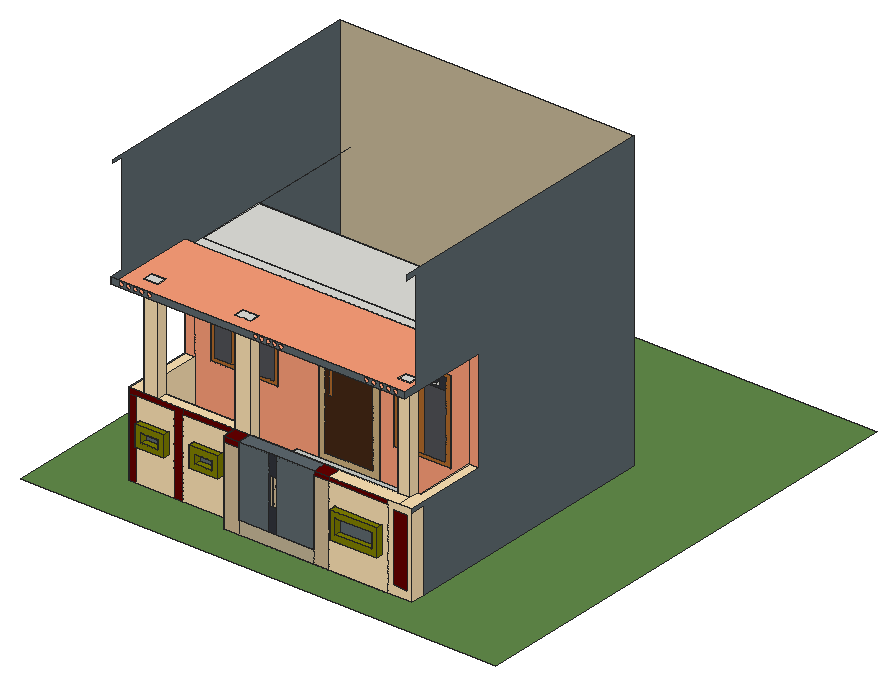
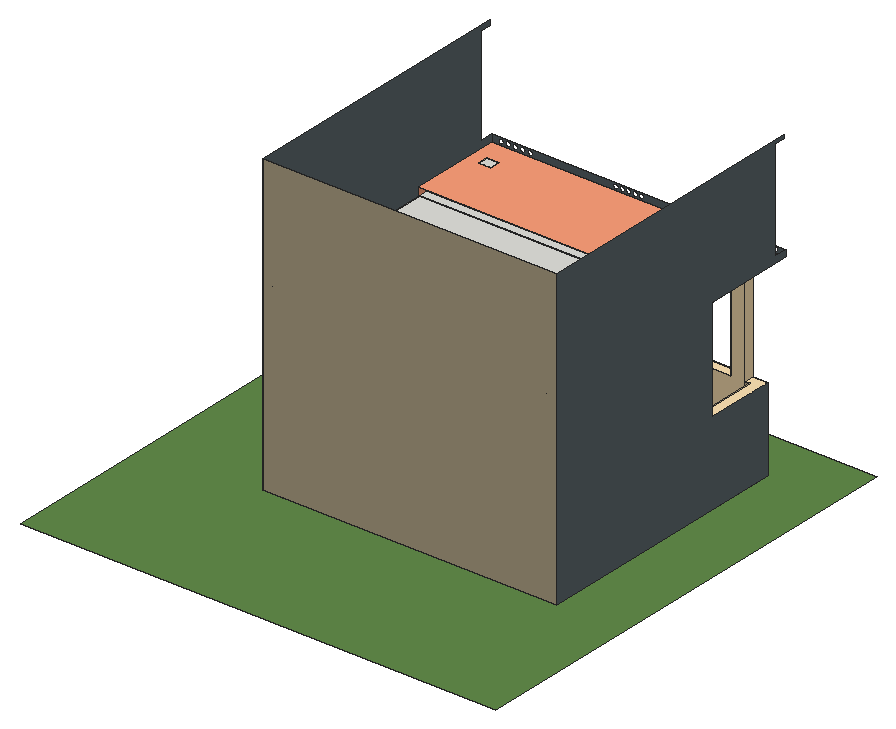
# SketchUp Ruby script. Lengths in inches.
U = 1.inch
M = Sketchup.active_model
def pt(a) = Geom::Point3d.new(a.map { |v| v * U })
def face(e, loops, mat)
  f = e.add_face(loops[0].map { |a| pt(a) })
  loops[1..].each { |l| e.add_face(l.map { |a| pt(a) }).erase! }
  f.material = f.back_material = mat if mat
  f
end
# faces: each face lists its corners as indices into pts; further lists are holes
def faces(e, pts, list, mat = nil) = list.each { |f| face(e, (f[0].is_a?(Array) ? f : [f]).map { |l| l.map { |i| pts[i] } }, mat) }
# xy, xz, yz: faces in a plane at the given z, y or x. An outline is a flat list of corners, or four numbers for a rectangle; further outlines are holes
def ring(l) = l.size == 4 ? [[l[0], l[1]], [l[2], l[1]], [l[2], l[3]], [l[0], l[3]]] : l.each_slice(2).to_a
def flat(e, list, mat, &to3) = list.each { |f| face(e, (f[0].is_a?(Array) ? f : [f]).map { |l| ring(l).map { |u, v| to3.(u, v) } }, mat) }
def xy(e, z, list, mat = nil) = flat(e, list, mat) { |x, y| [x, y, z] }
def xz(e, y, list, mat = nil) = flat(e, list, mat) { |x, z| [x, y, z] }
def yz(e, x, list, mat = nil) = flat(e, list, mat) { |y, z| [x, y, z] }
def lines(e, pts, list) = list.each { |a, b| e.add_line(pt(pts[a]), pt(pts[b])) }
# prism: a flat outline (further loops are holes) pulled along v
def prism(e, loops, v, mat = nil)
  f = face(e, loops, mat); d = Geom::Vector3d.new(v.map { |x| x * U })
  f.pushpull(f.normal.samedirection?(d) ? d.length : -d.length)
end
def box(e, o, s, mat = nil) = prism(e, [[o, [o[0] + s[0], o[1], o[2]], [o[0] + s[0], o[1] + s[1], o[2]], [o[0], o[1] + s[1], o[2]]]], [0, 0, s[2]], mat)
def at(x, y, z, deg = 0) = Geom::Transformation.translation(pt([x, y, z])) * Geom::Transformation.rotation(ORIGIN, Z_AXIS, deg.degrees)
def axes(o, x, y, z) = Geom::Transformation.new([*x, 0, *y, 0, *z, 0, *pt(o).to_a, 1])
def part(name) = M.definitions.add(name)
# library, detail: a bought-in or finely detailed component or shape, given as its bounding box
def library(name, o, s) = part(name).tap { |d| box(d.entities, o, s) }
def detail(e, o, s) = box(e.add_group.entities, o, s)
def put(e, d, t, mat = nil) = e.add_instance(d, t).tap { |i| i.material = mat if mat }
def group(e, t, mat = nil) = e.add_group.tap { |g| g.transformation = t; g.material = mat if mat }.entities
root = M.entities
M.materials.add("[0022_Maroon]").color = [128, 0, 0]
M.materials.add("[0026_LightSalmon]").color = [255, 160, 122]
M.materials.add("[0032_Moccasin]").color = [255, 228, 181]
M.materials.add("[0058_Olive]").color = [128, 128, 0]
M.materials.add("[Basic Tile]").color = [203, 206, 202]
M.materials.add("[Blinds Roman Hobbled Blue]").color = [81, 82, 87]
M.materials.add("[Carpet Berber Pattern Gray]").color = [165, 165, 165]
M.materials.add("[Color A08]").color = [102, 0, 0]
M.materials.add("[Color E08]").color = [102, 102, 0]
M.materials.add("[Formica Beige]").color = [211, 187, 149]
M.materials.add("[Formica Graystone]").color = [149, 146, 135]
M.materials.add("[Formica Laminate Dark]").color = [50, 53, 60]
M.materials.add("[Formica Speckled Grey]").color = [94, 105, 111]
M.materials.add("[Leather Blue]").color = [45, 57, 74]
M.materials.add("[Quartz Light Brown]").color = [199, 184, 152]
M.materials.add("[Terrazzo Light Blue]").color = [196, 214, 227]
M.materials.add("[Vegetation Grass Artificial]").color = [98, 140, 74]
M.materials.add("[Wood Bamboo]").color = [177, 105, 43]
M.materials.add("[Wood Floor Light]").color = [204, 176, 127]
M.materials.add("[Wood Veneer 01]").color = [68, 40, 21]
xy(root,0,[[120.55,26.1,120.55,35.67,47,35.67,47,218.93,251.02,218.93,251.02,35.67,233.76,35.67,233.76,26.1],[233.76,26.1,251.02,35.67]])
xy(root,0,[[0,0,330.1875,330.1875]],"[Vegetation Grass Artificial]")
xy(root,9,[[130.89,26.1,183.14,35.67],[53.84,91.2,244.18,139.9]])
xy(root,9,[[131.52,35.67,233.76,42.51]],"[Carpet Berber Pattern Gray]")
xy(root,9,[[53.84,42.51,244.18,42.51,244.18,84.33,199.57,84.33,199.57,53.64,124.76,53.64,124.76,84.33,53.84,84.33]],"[Leather Blue]")
xy(root,16.4375,[[124.76,53.64,199.57,63.72]],"[Basic Tile]")
xy(root,20.375,[[124.76,63.72,199.57,73.8]],"[Basic Tile]")
xy(root,22.07,[[197.18,21.79,230.37,26.1]],"[0058_Olive]")
xy(root,25.48,[[54.61,31.1,74.79,35.67],[91.98,31.1,112.17,35.67]],"[0058_Olive]")
xy(root,25.78,[[139.85,84.33,181.85,91.2]])
xy(root,25.78,[[124.76,73.8,199.57,84.33]],"[Basic Tile]")
xy(root,26.13,[[201.24,21.79,226.3,26.1]],"[0058_Olive]")
xy(root,29.55,[[58.67,31.1,70.73,35.67],[96.05,31.1,108.1,35.67]],"[0058_Olive]")
xy(root,35.79,[[58.67,31.1,70.73,35.67],[96.05,31.1,108.1,35.67]],"[0058_Olive]")
xy(root,36.69,[[201.24,21.79,226.3,26.1]],"[0058_Olive]")
xy(root,39.86,[[54.61,31.1,74.79,35.67],[91.98,31.1,112.17,35.67]],"[0058_Olive]")
xy(root,40.75,[[197.18,21.79,230.37,26.1]],"[0058_Olive]")
xy(root,50.11,[[192.03,84.33,231.1,91.2]])
xy(root,57.875,[[193.46,26.1,241.9375,35.67],[241.9375,26.1,251.02,26.1,251.02,84.33,244.18,84.33,244.18,42.51,241.9375,42.51],[47,35.67,56.97,35.67,56.97,42.51,53.84,42.51,53.84,84.33,47,84.33],[66.79,35.67,120.55,42.51]],"[0032_Moccasin]")
xy(root,57.875,[[120.55,26.1,130.89,35.67],[183.14,26.1,193.46,35.67]],"[Color A08]")
xy(root,57.875,[[130.89,26.1,183.14,35.67]],"[Formica Speckled Grey]")
xy(root,59.35,[[64.57,84.33,111.51,91.2]])
xy(root,109.17,[[192.03,84.33,231.1,91.2]])
xy(root,113.17,[[64.57,84.33,111.51,91.2]])
xy(root,119.59,[[139.85,84.33,181.85,91.2]])
xy(root,129,[[56.97,35.67,66.79,42.51],[120.55,35.67,131.52,42.51],[233.76,35.67,241.9375,42.51],[53.84,84.33,244.18,91.2],[53.84,91.2,244.18,139.9]])
xy(root,129,[[[47,20.01,251.02,84.33],[120.55,35.67,131.52,42.51],[56.97,35.67,66.79,42.51],[233.76,35.67,241.9375,42.51]]],"[0026_LightSalmon]")
xz(root,20.01,[[[47,129,251.02,133.625],[244.56,129.67,244.09,129.73,243.65,129.91,243.28,130.2,242.99,130.57,242.81,131.01,242.75,131.48,242.81,131.95,242.99,132.38,243.28,132.76,243.65,133.05,244.09,133.23,244.56,133.29,245.03,133.23,245.47,133.05,245.84,132.76,246.13,132.38,246.3125,131.95,246.37,131.48,246.3125,131.01,246.13,130.57,245.84,130.2,245.47,129.91,245.03,129.73],[239.62,129.67,239.15,129.73,238.72,129.91,238.34,130.2,238.05,130.57,237.87,131.01,237.81,131.48,237.87,131.95,238.05,132.38,238.34,132.76,238.72,133.05,239.15,133.23,239.62,133.29,240.09,133.23,240.53,133.05,240.9,132.76,241.19,132.38,241.375,131.95,241.44,131.48,241.375,131.01,241.19,130.57,240.9,130.2,240.53,129.91,240.09,129.73],[234.56,129.67,234.09,129.73,233.65,129.91,233.28,130.2,232.99,130.57,232.81,131.01,232.75,131.48,232.81,131.95,232.99,132.38,233.28,132.76,233.65,133.05,234.09,133.23,234.56,133.29,235.03,133.23,235.47,133.05,235.84,132.76,236.13,132.38,236.3125,131.95,236.37,131.48,236.3125,131.01,236.13,130.57,235.84,130.2,235.47,129.91,235.03,129.73],[229.44,129.67,228.97,129.73,228.53,129.91,228.15,130.2,227.87,130.57,227.68,131.01,227.62,131.48,227.68,131.95,227.87,132.38,228.15,132.76,228.53,133.05,228.97,133.23,229.44,133.29,229.9,133.23,230.34,133.05,230.72,132.76,231,132.38,231.1875,131.95,231.25,131.48,231.1875,131.01,231,130.57,230.72,130.2,230.34,129.91,229.9,129.73],[224.19,129.67,223.72,129.73,223.28,129.91,222.9,130.2,222.62,130.57,222.43,131.01,222.37,131.48,222.43,131.95,222.62,132.38,222.9,132.76,223.28,133.05,223.72,133.23,224.19,133.29,224.65,133.23,225.09,133.05,225.47,132.76,225.75,132.38,225.9375,131.95,226,131.48,225.9375,131.01,225.75,130.57,225.47,130.2,225.09,129.91,224.65,129.73],[58.94,129.67,58.47,129.73,58.03,129.91,57.65,130.2,57.37,130.57,57.18,131.01,57.12,131.48,57.18,131.95,57.37,132.38,57.65,132.76,58.03,133.05,58.47,133.23,58.94,133.29,59.4,133.23,59.84,133.05,60.22,132.76,60.5,132.38,60.6875,131.95,60.75,131.48,60.6875,131.01,60.5,130.57,60.22,130.2,59.84,129.91,59.4,129.73],[63.56,129.67,63.09,129.73,62.65,129.91,62.28,130.2,61.99,130.57,61.81,131.01,61.75,131.48,61.81,131.95,61.99,132.38,62.28,132.76,62.65,133.05,63.09,133.23,63.56,133.29,64.03,133.23,64.47,133.05,64.84,132.76,65.13,132.38,65.3125,131.95,65.37,131.48,65.3125,131.01,65.13,130.57,64.84,130.2,64.47,129.91,64.03,129.73],[68.31,129.67,67.84,129.73,67.4,129.91,67.03,130.2,66.74,130.57,66.56,131.01,66.5,131.48,66.56,131.95,66.74,132.38,67.03,132.76,67.4,133.05,67.84,133.23,68.31,133.29,68.78,133.23,69.22,133.05,69.59,132.76,69.88,132.38,70.0625,131.95,70.12,131.48,70.0625,131.01,69.88,130.57,69.59,130.2,69.22,129.91,68.78,129.73],[73.62,129.67,73.15,129.73,72.72,129.91,72.34,130.2,72.05,130.57,71.87,131.01,71.81,131.48,71.87,131.95,72.05,132.38,72.34,132.76,72.72,133.05,73.15,133.23,73.62,133.29,74.09,133.23,74.53,133.05,74.9,132.76,75.19,132.38,75.375,131.95,75.44,131.48,75.375,131.01,75.19,130.57,74.9,130.2,74.53,129.91,74.09,129.73],[147.06,129.67,146.59,129.73,146.15,129.91,145.78,130.2,145.49,130.57,145.31,131.01,145.25,131.48,145.31,131.95,145.49,132.38,145.78,132.76,146.15,133.05,146.59,133.23,147.06,133.29,147.53,133.23,147.97,133.05,148.34,132.76,148.63,132.38,148.8125,131.95,148.87,131.48,148.8125,131.01,148.63,130.57,148.34,130.2,147.97,129.91,147.53,129.73],[151.44,129.67,150.97,129.73,150.53,129.91,150.15,130.2,149.87,130.57,149.68,131.01,149.62,131.48,149.68,131.95,149.87,132.38,150.15,132.76,150.53,133.05,150.97,133.23,151.44,133.29,151.9,133.23,152.34,133.05,152.72,132.76,153,132.38,153.1875,131.95,153.25,131.48,153.1875,131.01,153,130.57,152.72,130.2,152.34,129.91,151.9,129.73],[156,129.67,155.53,129.73,155.09,129.91,154.72,130.2,154.43,130.57,154.25,131.01,154.19,131.48,154.25,131.95,154.43,132.38,154.72,132.76,155.09,133.05,155.53,133.23,156,133.29,156.47,133.23,156.9,133.05,157.28,132.76,157.57,132.38,157.75,131.95,157.81,131.48,157.75,131.01,157.57,130.57,157.28,130.2,156.9,129.91,156.47,129.73],[160.31,129.67,159.84,129.73,159.4,129.91,159.03,130.2,158.74,130.57,158.56,131.01,158.5,131.48,158.56,131.95,158.74,132.38,159.03,132.76,159.4,133.05,159.84,133.23,160.31,133.29,160.78,133.23,161.22,133.05,161.59,132.76,161.88,132.38,162.0625,131.95,162.12,131.48,162.0625,131.01,161.88,130.57,161.59,130.2,161.22,129.91,160.78,129.73],[164.87,129.67,164.4,129.73,163.97,129.91,163.59,130.2,163.3,130.57,163.12,131.01,163.06,131.48,163.12,131.95,163.3,132.38,163.59,132.76,163.97,133.05,164.4,133.23,164.87,133.29,165.34,133.23,165.78,133.05,166.15,132.76,166.44,132.38,166.625,131.95,166.69,131.48,166.625,131.01,166.44,130.57,166.15,130.2,165.78,129.91,165.34,129.73],[54,129.67,53.53,129.73,53.09,129.91,52.72,130.2,52.43,130.57,52.25,131.01,52.19,131.48,52.25,131.95,52.43,132.38,52.72,132.76,53.09,133.05,53.53,133.23,54,133.29,54.47,133.23,54.9,133.05,55.28,132.76,55.57,132.38,55.75,131.95,55.81,131.48,55.75,131.01,55.57,130.57,55.28,130.2,54.9,129.91,54.47,129.73]]],"[Formica Speckled Grey]")
xz(root,21.79,[[[197.18,22.07,230.37,40.75],[201.24,26.13,226.3,36.69]]],"[0058_Olive]")
xz(root,26.1,[[[193.46,0,234.59,54.98],[197.18,22.07,230.37,40.75]],[[234.59,0,251.02,57.875],[237.47,5.84,248.4,53.15]]],"[0032_Moccasin]")
xz(root,26.1,[[237.47,5.84,248.4,53.15],[120.55,53.96,130.89,57.875],[183.14,54.98,193.46,57.875],[193.46,54.98,234.59,57.875]],"[Color A08]")
xz(root,26.1,[[120.55,0,130.89,53.96],[183.14,0,193.46,54.98],[152.71,25.63,154.02,43.88],[155.02,25.63,156.34,43.88]],"[Formica Beige]")
xz(root,26.1,[[[151.42,9,157.36,57.875],[152.71,25.63,154.02,43.88],[155.02,25.63,156.34,43.88]]],"[Formica Laminate Dark]")
xz(root,26.1,[[130.89,9,151.42,57.875],[157.36,9,183.14,57.875],[201.24,26.13,226.3,36.69]],"[Formica Speckled Grey]")
xz(root,26.1,[[130.89,0,183.14,9]],"[Quartz Light Brown]")
xz(root,31.1,[[[54.61,25.48,74.79,39.86],[58.67,29.55,70.73,35.79]],[[91.98,25.48,112.17,39.86],[96.05,29.55,108.1,35.79]]],"[0058_Olive]")
xz(root,35.67,[[233.76,0,251.02,54.98],[130.89,9,131.52,57.875]])
xz(root,35.67,[[[51.625,0,78.15,53.96],[54.61,25.48,74.79,39.86]],[[84.45,0,120.55,53.96],[91.98,25.48,112.17,39.86]],[183.14,9,233.76,54.98],[183.14,54.98,233.76,57.875],[56.97,57.875,66.79,129],
  [120.55,57.875,131.52,129],[233.76,57.875,241.9375,129]],"[0032_Moccasin]")
xz(root,35.67,[[47,0,51.625,53.96],[78.15,0,84.45,0,84.45,57.875,47,57.875,47,53.96,78.15,53.96],[84.45,53.96,120.55,57.875]],"[Color A08]")
xz(root,35.67,[[131.52,9,183.14,57.875],[58.67,29.55,70.73,35.79],[96.05,29.55,108.1,35.79]],"[Formica Speckled Grey]")
xz(root,42.51,[[56.97,9,56.97,129,66.79,129,66.79,57.875,120.55,57.875,120.55,9],[120.55,9,131.52,129],[233.76,9,241.9375,129]],"[0032_Moccasin]")
xz(root,42.51,[[53.84,9,56.97,57.875],[241.9375,9,244.18,57.875]],"[Formica Beige]")
xz(root,53.64,[[124.76,9,199.57,16.4375]],"[Terrazzo Light Blue]")
xz(root,63.72,[[124.76,16.4375,199.57,20.375]],"[Basic Tile]")
xz(root,73.8,[[124.76,20.375,199.57,25.78]],"[Basic Tile]")
xz(root,84.33,[[[200.51,98.74,201.34,98.78,202.13,99.03,202.83,99.48,203.39,100.1,203.77,100.84,203.95,101.65,203.91,102.48,203.65,103.28,203.2,103.97,202.59,104.53,201.85,104.92,201.04,105.09,200.2,105.05,199.41,104.8,198.71,104.35,198.15,103.73,197.77,102.99,197.6,102.18,197.64,101.35,197.89,100.55,198.34,99.85,198.96,99.3,199.7,98.91],[200.61,100,200.125,100.11,199.68,100.34,199.31,100.67,199.04,101.1,198.88,101.57,198.86,102.07,198.96,102.5625,199.19,103.01,199.53,103.38,199.95,103.65,200.43,103.8,200.93,103.83,201.42,103.72,201.87,103.49,202.24,103.16,202.51,102.73,202.66,102.26,202.6875,101.76,202.58,101.27,202.35,100.82,202.01,100.45,201.59,100.18,201.11,100.03]],[[210.2,98.74,211.03,98.78,211.82,99.03,212.52,99.48,213.08,100.1,213.46,100.84,213.64,101.65,213.6,102.48,213.34,103.28,212.89,103.97,212.28,104.53,211.54,104.92,210.72,105.09,209.89,105.05,209.1,104.8,208.4,104.35,207.84,103.73,207.46,102.99,207.28,102.18,207.32,101.35,207.58,100.55,208.03,99.85,208.64,99.3,209.38,98.91],[210.3,100,209.8125,100.11,209.37,100.34,208.99,100.67,208.72,101.1,208.57,101.57,208.55,102.07,208.65,102.5625,208.88,103.01,209.22,103.38,209.64,103.65,210.12,103.8,210.62,103.83,211.11,103.72,211.55,103.49,211.93,103.16,212.2,102.73,212.35,102.26,212.375,101.76,212.27,101.27,212.04,100.82,211.7,100.45,211.28,100.18,210.8,100.03]],[[220.7,98.74,221.53,98.78,222.32,99.03,223.02,99.48,223.58,100.1,223.96,100.84,224.14,101.65,224.1,102.48,223.84,103.28,223.39,103.97,222.78,104.53,222.04,104.92,221.22,105.09,220.39,105.05,219.6,104.8,218.9,104.35,218.34,103.73,217.96,102.99,217.78,102.18,217.82,101.35,218.08,100.55,218.53,99.85,219.14,99.3,219.88,98.91],[220.8,100,220.3125,100.11,219.87,100.34,219.49,100.67,219.22,101.1,219.07,101.57,219.05,102.07,219.15,102.5625,219.38,103.01,219.72,103.38,220.14,103.65,220.62,103.8,221.12,103.83,221.61,103.72,222.05,103.49,222.43,103.16,222.7,102.73,222.85,102.26,222.875,101.76,222.77,101.27,222.54,100.82,222.2,100.45,221.78,100.18,221.3,100.03]],[[75.4,103.07,76.23,103.11,77.02,103.37,77.72,103.82,78.28,104.43,78.66,105.17,78.84,105.99,78.8,106.82,78.54,107.61,78.09,108.31,77.48,108.87,76.74,109.25,75.92,109.43,75.09,109.39,74.3,109.13,73.6,108.68,73.04,108.07,72.66,107.33,72.48,106.51,72.52,105.68,72.78,104.89,73.23,104.1875,73.84,103.63,74.58,103.25],[75.5,104.34,75.01,104.44,74.57,104.67,74.19,105.01,73.92,105.43,73.77,105.91,73.75,106.41,73.85,106.9,74.08,107.34,74.42,107.71,74.84,107.99,75.32,108.14,75.82,108.16,76.31,108.06,76.75,107.83,77.125,107.49,77.4,107.07,77.55,106.59,77.57,106.09,77.47,105.6,77.24,105.15,76.9,104.78,76.48,104.51,76,104.36]],[[86.46,103.07,87.29,103.11,88.08,103.37,88.78,103.82,89.34,104.43,89.72,105.17,89.9,105.99,89.86,106.82,89.6,107.61,89.15,108.31,88.54,108.87,87.8,109.25,86.99,109.43,86.15,109.39,85.36,109.13,84.66,108.68,84.1,108.07,83.72,107.33,83.55,106.51,83.59,105.68,83.84,104.89,84.29,104.1875,84.91,103.63,85.65,103.25],[86.5625,104.34,86.07,104.44,85.63,104.67,85.26,105.01,84.99,105.43,84.83,105.91,84.81,106.41,84.91,106.9,85.14,107.34,85.48,107.71,85.9,107.99,86.38,108.14,86.88,108.16,87.37,108.06,87.82,107.83,88.1875,107.49,88.46,107.07,88.61,106.59,88.64,106.09,88.53,105.6,88.3,105.15,87.96,104.78,87.54,104.51,87.0625,104.36]],
  [[99.77,103.07,100.6,103.11,101.4,103.37,102.09,103.82,102.65,104.43,103.04,105.17,103.21,105.99,103.17,106.82,102.92,107.61,102.47,108.31,101.85,108.87,101.11,109.25,100.3,109.43,99.47,109.39,98.67,109.13,97.97,108.68,97.42,108.07,97.03,107.33,96.86,106.51,96.9,105.68,97.15,104.89,97.6,104.1875,98.22,103.63,98.96,103.25],[99.875,104.34,99.39,104.44,98.94,104.67,98.57,105.01,98.3,105.43,98.14,105.91,98.12,106.41,98.23,106.9,98.46,107.34,98.79,107.71,99.22,107.99,99.69,108.14,100.19,108.16,100.68,108.06,101.13,107.83,101.5,107.49,101.77,107.07,101.92,106.59,101.95,106.09,101.84,105.6,101.61,105.15,101.28,104.78,100.85,104.51,100.375,104.36]]])
xz(root,84.33,[[[53.84,9,124.76,9,124.76,25.78,139.85,25.78,139.85,119.59,181.85,119.59,181.85,25.78,199.57,25.78,199.57,9,244.18,9,244.18,129,53.84,129],[64.57,59.35,111.51,113.17],[192.03,50.11,231.1,109.17]],[47,57.875,53.84,129],[244.18,57.875,251.02,129]],"[0026_LightSalmon]")
xz(root,84.33,[[195.21,53.29,209.06,98.1],[212.94,53.29,227.92,98.1],[67.35,62.13,78.72,101.66],[81.26,62.13,93.32,101.66],[95.69,62.13,108.73,101.66]],"[Blinds Roman Hobbled Blue]")
xz(root,84.33,[[[195.21,98.1,227.92,105.99],[200.51,98.74,199.7,98.91,198.96,99.3,198.34,99.85,197.89,100.55,197.64,101.35,197.6,102.18,197.77,102.99,198.15,103.73,198.71,104.35,199.41,104.8,200.2,105.05,201.04,105.09,201.85,104.92,202.59,104.53,203.2,103.97,203.65,103.28,203.91,102.48,203.95,101.65,203.77,100.84,203.39,100.1,202.83,99.48,202.13,99.03,201.34,98.78],[220.7,98.74,219.88,98.91,219.14,99.3,218.53,99.85,218.08,100.55,217.82,101.35,217.78,102.18,217.96,102.99,218.34,103.73,218.9,104.35,219.6,104.8,220.39,105.05,221.22,105.09,222.04,104.92,222.78,104.53,223.39,103.97,223.84,103.28,224.1,102.48,224.14,101.65,223.96,100.84,223.58,100.1,223.02,99.48,222.32,99.03,221.53,98.78],[210.2,98.74,209.38,98.91,208.64,99.3,208.03,99.85,207.58,100.55,207.32,101.35,207.28,102.18,207.46,102.99,207.84,103.73,208.4,104.35,209.1,104.8,209.89,105.05,210.72,105.09,211.54,104.92,212.28,104.53,212.89,103.97,213.34,103.28,213.6,102.48,213.64,101.65,213.46,100.84,213.08,100.1,212.52,99.48,211.82,99.03,211.03,98.78]],[200.61,100,201.11,100.03,201.59,100.18,202.01,100.45,202.35,100.82,202.58,101.27,202.6875,101.76,202.66,102.26,202.51,102.73,202.24,103.16,201.87,103.49,201.42,103.72,200.93,103.83,200.43,103.8,199.95,103.65,199.53,103.38,199.19,103.01,198.96,102.5625,198.86,102.07,198.88,101.57,199.04,101.1,199.31,100.67,199.68,100.34,200.125,100.11],[210.3,100,210.8,100.03,211.28,100.18,211.7,100.45,212.04,100.82,212.27,101.27,212.375,101.76,212.35,102.26,212.2,102.73,211.93,103.16,211.55,103.49,211.11,103.72,210.62,103.83,210.12,103.8,209.64,103.65,209.22,103.38,208.88,103.01,208.65,102.5625,208.55,102.07,208.57,101.57,208.72,101.1,208.99,100.67,209.37,100.34,209.8125,100.11],[220.8,100,221.3,100.03,221.78,100.18,222.2,100.45,222.54,100.82,222.77,101.27,222.875,101.76,222.85,102.26,222.7,102.73,222.43,103.16,222.05,103.49,221.61,103.72,221.12,103.83,220.62,103.8,220.14,103.65,219.72,103.38,219.38,103.01,219.15,102.5625,219.05,102.07,219.07,101.57,219.22,101.1,219.49,100.67,219.87,100.34,220.3125,100.11],[[67.35,101.66,108.73,110.39],[75.4,103.07,74.58,103.25,73.84,103.63,73.23,104.1875,72.78,104.89,72.52,105.68,72.48,106.51,72.66,107.33,73.04,108.07,73.6,108.68,74.3,109.13,75.09,109.39,75.92,109.43,76.74,109.25,77.48,108.87,78.09,108.31,78.54,107.61,78.8,106.82,78.84,105.99,78.66,105.17,78.28,104.43,77.72,103.82,77.02,103.37,76.23,103.11],[99.77,103.07,98.96,103.25,98.22,103.63,97.6,104.1875,97.15,104.89,96.9,105.68,96.86,106.51,97.03,107.33,97.42,108.07,97.97,108.68,98.67,109.13,99.47,109.39,100.3,109.43,101.11,109.25,101.85,108.87,102.47,108.31,102.92,107.61,103.17,106.82,103.21,105.99,103.04,105.17,102.65,104.43,102.09,103.82,101.4,103.37,100.6,103.11],[86.46,103.07,85.65,103.25,84.91,103.63,84.29,104.1875,83.84,104.89,83.59,105.68,83.55,106.51,83.72,107.33,84.1,108.07,84.66,108.68,85.36,109.13,86.15,109.39,86.99,109.43,87.8,109.25,88.54,108.87,89.15,108.31,89.6,107.61,89.86,106.82,89.9,105.99,89.72,105.17,89.34,104.43,88.78,103.82,88.08,103.37,87.29,103.11]],
  [75.5,104.34,76,104.36,76.48,104.51,76.9,104.78,77.24,105.15,77.47,105.6,77.57,106.09,77.55,106.59,77.4,107.07,77.125,107.49,76.75,107.83,76.31,108.06,75.82,108.16,75.32,108.14,74.84,107.99,74.42,107.71,74.08,107.34,73.85,106.9,73.75,106.41,73.77,105.91,73.92,105.43,74.19,105.01,74.57,104.67,75.01,104.44],[86.5625,104.34,87.0625,104.36,87.54,104.51,87.96,104.78,88.3,105.15,88.53,105.6,88.64,106.09,88.61,106.59,88.46,107.07,88.1875,107.49,87.82,107.83,87.37,108.06,86.88,108.16,86.38,108.14,85.9,107.99,85.48,107.71,85.14,107.34,84.91,106.9,84.81,106.41,84.83,105.91,84.99,105.43,85.26,105.01,85.63,104.67,86.07,104.44],[99.875,104.34,100.375,104.36,100.85,104.51,101.28,104.78,101.61,105.15,101.84,105.6,101.95,106.09,101.92,106.59,101.77,107.07,101.5,107.49,101.13,107.83,100.68,108.06,100.19,108.16,99.69,108.14,99.22,107.99,98.79,107.71,98.46,107.34,98.23,106.9,98.12,106.41,98.14,105.91,98.3,105.43,98.57,105.01,98.94,104.67,99.39,104.44]],"[Formica Laminate Dark]")
xz(root,84.33,[[[192.03,50.11,231.1,109.17],[195.21,53.29,227.92,105.99]],[209.06,53.29,212.94,98.1],[[64.57,59.35,111.51,113.17],[67.35,62.13,108.73,110.39]],[78.72,62.13,81.26,101.66],[93.32,62.13,95.69,101.66],
  [146.87,66.47,149.37,85.72]],"[Wood Bamboo]")
xz(root,84.33,[[[139.85,25.78,181.85,119.59],[144.16,30.08,177.55,115.29]],[144.16,105.375,177.55,108.49]],"[Wood Floor Light]")
xz(root,84.33,[[[144.16,30.08,177.55,105.375],[146.87,66.47,149.37,85.72]],[144.16,108.49,177.55,115.29]],"[Wood Veneer 01]")
xz(root,91.2,[[[53.84,9,244.18,129],[139.85,25.78,181.85,119.59],[64.57,59.35,111.51,113.17],[192.03,50.11,231.1,109.17]]])
xz(root,139.9,[[53.84,9,244.18,129]],"[Formica Graystone]")
xz(root,218.93,[[47,0,251.02,205.625]],"[Quartz Light Brown]")
yz(root,47,[[35.67,0,35.67,57.875,84.33,57.875,84.33,129,20.01,129,20.01,133.625,29.17,133.625,29.17,203.49,21.86,203.49,21.86,205.625,218.93,205.625,218.93,0]],"[Formica Speckled Grey]")
yz(root,53.84,[[91.2,9,139.9,129]])
yz(root,53.84,[[42.51,9,84.33,57.875]],"[0032_Moccasin]")
yz(root,54.61,[[31.1,25.48,35.67,39.86]],"[0058_Olive]")
yz(root,56.97,[[35.67,57.875,42.51,129]],"[0032_Moccasin]")
yz(root,58.67,[[31.1,29.55,35.67,35.79]],"[0058_Olive]")
yz(root,64.57,[[84.33,59.35,91.2,113.17]])
yz(root,66.79,[[35.67,57.875,42.51,129]],"[0032_Moccasin]")
yz(root,70.73,[[31.1,29.55,35.67,35.79]],"[0058_Olive]")
yz(root,74.79,[[31.1,25.48,35.67,39.86]],"[0058_Olive]")
yz(root,91.98,[[31.1,25.48,35.67,39.86]],"[0058_Olive]")
yz(root,96.05,[[31.1,29.55,35.67,35.79]],"[0058_Olive]")
yz(root,108.1,[[31.1,29.55,35.67,35.79]],"[0058_Olive]")
yz(root,111.51,[[84.33,59.35,91.2,113.17]])
yz(root,112.17,[[31.1,25.48,35.67,39.86]],"[0058_Olive]")
yz(root,120.55,[[26.1,53.96,35.67,57.875]],"[0022_Maroon]")
yz(root,120.55,[[26.1,0,35.67,53.96],[35.67,57.875,42.51,129]],"[0032_Moccasin]")
yz(root,124.76,[[53.64,9,63.72,16.4375],[63.72,9,73.8,20.375],[73.8,9,84.33,25.78]],"[Basic Tile]")
yz(root,130.89,[[26.1,9,35.67,57.875]])
yz(root,131.52,[[35.67,9,42.51,129]],"[0032_Moccasin]")
yz(root,139.85,[[84.33,25.78,91.2,119.59]])
yz(root,181.85,[[84.33,25.78,91.2,119.59]])
yz(root,183.14,[[26.1,9,35.67,54.98]])
yz(root,192.03,[[84.33,50.11,91.2,109.17]])
yz(root,197.18,[[21.79,22.07,26.1,40.75]],"[Color E08]")
yz(root,199.57,[[53.64,9,63.72,16.4375],[63.72,9,73.8,20.375],[73.8,9,84.33,25.78]],"[Basic Tile]")
yz(root,201.24,[[21.79,26.13,26.1,36.69]],"[0058_Olive]")
yz(root,226.3,[[21.79,26.13,26.1,36.69]],"[0058_Olive]")
yz(root,230.37,[[21.79,22.07,26.1,40.75]],"[0058_Olive]")
yz(root,231.1,[[84.33,50.11,91.2,109.17]])
yz(root,233.76,[[35.67,9,42.51,129]],"[0032_Moccasin]")
yz(root,241.9375,[[35.67,57.875,42.51,129]],"[0032_Moccasin]")
yz(root,244.18,[[91.2,9,139.9,129]])
yz(root,244.18,[[42.51,9,84.33,57.875]],"[0032_Moccasin]")
yz(root,251.02,[[26.1,0,35.67,54.98]],"[0032_Moccasin]")
yz(root,251.02,[[35.67,0,218.93,0,218.93,205.625,21.86,205.625,21.86,202.04,29.17,202.04,29.17,133.625,20.01,133.625,20.01,129,84.33,129,84.33,57.875,26.1,57.875,26.1,54.98,35.67,54.98]],"[Formica Speckled Grey]")
p = [[53.84,139.9,129],[53.84,218.93,129],[244.18,139.9,129],[244.18,218.93,129],[233.76,35.67,9],[233.76,26.1,9]]
lines(root,p,[[0,1],[2,3],[4,5]])
